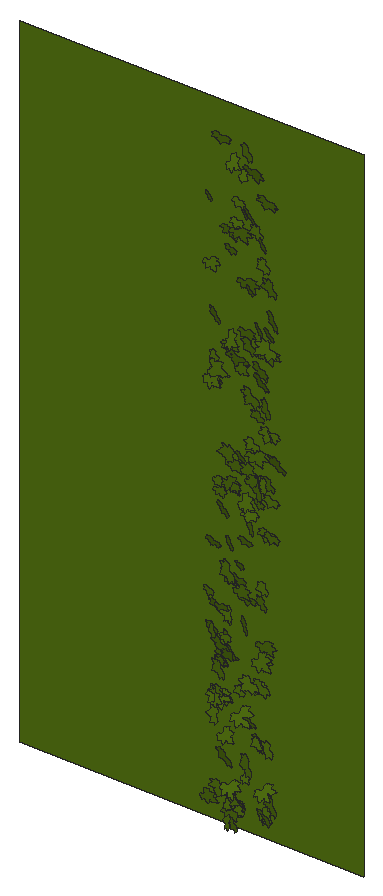
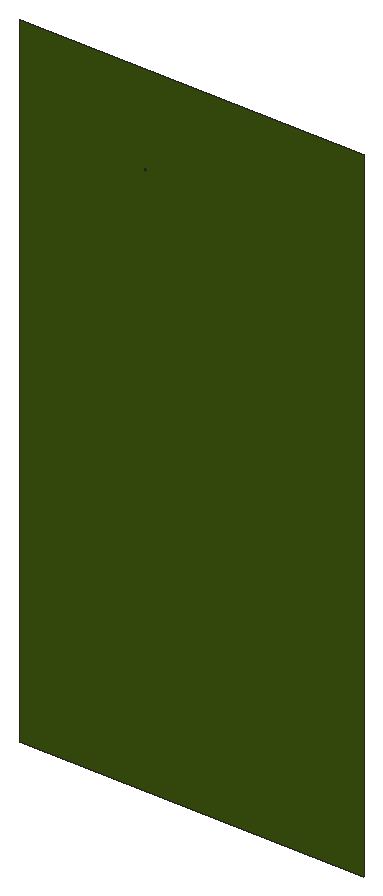
# SketchUp Ruby script. Lengths in inches.
U = 1.inch
M = Sketchup.active_model
def pt(a) = Geom::Point3d.new(a.map { |v| v * U })
def face(e, loops, mat)
  f = e.add_face(loops[0].map { |a| pt(a) })
  loops[1..].each { |l| e.add_face(l.map { |a| pt(a) }).erase! }
  f.material = f.back_material = mat if mat
  f
end
# faces: each face lists its corners as indices into pts; further lists are holes
def faces(e, pts, list, mat = nil) = list.each { |f| face(e, (f[0].is_a?(Array) ? f : [f]).map { |l| l.map { |i| pts[i] } }, mat) }
# xy, xz, yz: faces in a plane at the given z, y or x. An outline is a flat list of corners, or four numbers for a rectangle; further outlines are holes
def ring(l) = l.size == 4 ? [[l[0], l[1]], [l[2], l[1]], [l[2], l[3]], [l[0], l[3]]] : l.each_slice(2).to_a
def flat(e, list, mat, &to3) = list.each { |f| face(e, (f[0].is_a?(Array) ? f : [f]).map { |l| ring(l).map { |u, v| to3.(u, v) } }, mat) }
def xy(e, z, list, mat = nil) = flat(e, list, mat) { |x, y| [x, y, z] }
def xz(e, y, list, mat = nil) = flat(e, list, mat) { |x, z| [x, y, z] }
def yz(e, x, list, mat = nil) = flat(e, list, mat) { |y, z| [x, y, z] }
def lines(e, pts, list) = list.each { |a, b| e.add_line(pt(pts[a]), pt(pts[b])) }
# prism: a flat outline (further loops are holes) pulled along v
def prism(e, loops, v, mat = nil)
  f = face(e, loops, mat); d = Geom::Vector3d.new(v.map { |x| x * U })
  f.pushpull(f.normal.samedirection?(d) ? d.length : -d.length)
end
def box(e, o, s, mat = nil) = prism(e, [[o, [o[0] + s[0], o[1], o[2]], [o[0] + s[0], o[1] + s[1], o[2]], [o[0], o[1] + s[1], o[2]]]], [0, 0, s[2]], mat)
def at(x, y, z, deg = 0) = Geom::Transformation.translation(pt([x, y, z])) * Geom::Transformation.rotation(ORIGIN, Z_AXIS, deg.degrees)
def axes(o, x, y, z) = Geom::Transformation.new([*x, 0, *y, 0, *z, 0, *pt(o).to_a, 1])
def part(name) = M.definitions.add(name)
# library, detail: a bought-in or finely detailed component or shape, given as its bounding box
def library(name, o, s) = part(name).tap { |d| box(d.entities, o, s) }
def detail(e, o, s) = box(e.add_group.entities, o, s)
def put(e, d, t, mat = nil) = e.add_instance(d, t).tap { |i| i.material = mat if mat }
def group(e, t, mat = nil) = e.add_group.tap { |g| g.transformation = t; g.material = mat if mat }.entities
root = M.entities
M.materials.add("[Vegetation Blur 03]").color = [83, 114, 18]
c1 = part("ivy")
xy(c1.entities,0,[[0.782,0,0.786,0,0.787,0.005,0.789,0.009,0.821,0.072,0.875,0.147,1.001,0.272,1.073,0.331,1.137,0.363,1.178,0.379,1.223,0.384,1.272,0.383,1.311,0.374,1.36,0.355,1.399,0.334,1.491,0.285,1.541,0.244,1.583,0.199,1.617,0.15,1.64,0.128,1.662,0.115,1.717,0.105,1.745,0.093,1.784,0.054,1.819,0.057,1.854,0.064,1.882,0.075,1.896,0.074,1.91,0.071,1.937,0.063,1.964,0.053,1.99,0.038,2.016,0.015,2.034,0.002,2.04,0,2.038,0.003,2.036,0.007,2.033,0.038,2.036,0.068,2.045,0.1,2.055,0.116,2.064,0.123,2.077,0.129,2.088,0.129,2.106,0.132,2.118,0.13,2.179,0.132,2.207,0.133,2.225,0.133,2.242,0.138,2.22,0.162,2.207,0.186,2.206,0.213,2.212,0.236,2.228,0.262,2.247,0.274,2.298,0.283,2.355,0.294,2.37,0.296,2.376,0.295,2.377,0.3,2.377,0.303,2.385,0.329,2.411,0.37,2.426,0.392,2.449,0.407,2.511,0.426,2.561,0.444,2.619,0.466,2.589,0.469,2.561,0.476,2.501,0.5,2.449,0.516,2.424,0.523,2.401,0.535,2.377,0.556,2.372,0.568,2.36,0.575,2.268,0.586,2.225,0.592,2.207,0.599,2.194,0.61,2.143,0.65,2.13,0.664,2.122,0.682,2.123,0.7,2.13,0.719,2.148,0.75,2.17,0.781,2.195,0.807,2.221,0.828,2.284,0.874,2.291,0.88,2.288,0.887,2.276,0.9,2.267,0.916,2.265,0.933,2.273,0.967,2.292,1.002,2.313,1.03,2.334,1.054,2.348,1.067,2.358,1.074,2.363,1.076,2.362,1.081,2.35,1.094,2.347,1.11,2.35,1.143,2.359,1.18,2.385,1.254,2.415,1.324,2.448,1.393,2.45,1.4,2.446,1.398,2.44,1.394,2.427,1.383,2.402,1.36,2.376,1.339,2.345,1.324,2.305,1.309,2.282,1.303,2.273,1.306,2.245,1.294,2.212,1.287,2.187,1.291,2.163,1.301,2.142,1.316,2.134,1.327,2.124,1.325,2.09,1.292,2.053,1.259,2.014,1.234,1.973,1.215,1.954,1.21,1.931,1.208,1.909,1.212,1.893,1.22,1.879,1.233,1.872,1.248,1.867,1.281,1.864,1.319,1.821,1.258,1.773,1.197,1.726,1.141,1.698,1.121,1.679,1.116,1.666,1.117,1.647,1.122,1.632,1.129,1.62,1.141,1.617,1.154,1.617,1.219,1.621,1.254,1.623,1.268,1.623,1.281,1.618,1.314,1.606,1.346,1.603,1.375,1.607,1.403,1.603,1.467,1.599,1.499,1.605,1.525,1.614,1.552,1.629,1.577,1.635,1.589,1.629,1.587,1.618,1.582,1.596,1.566,1.581,1.556,1.568,1.552,1.557,1.55,1.545,1.553,1.531,1.562,1.522,1.572,1.504,1.591,1.486,1.611,1.474,1.631,1.457,1.666,1.455,1.684,1.457,1.698,1.452,1.715,1.444,1.728,1.424,1.754,1.419,1.772,1.423,1.786,1.434,1.819,1.444,1.848,1.446,1.855,1.44,1.861,1.43,1.867,1.386,1.904,1.349,1.948,1.326,1.973,1.31,1.995,1.288,2.048,1.284,2.153,1.287,2.254,1.284,2.255,1.282,2.253,1.278,2.247,1.274,2.237,1.266,2.216,1.226,2.125,1.208,2.076,1.184,2.033,1.155,1.984,1.135,1.942,1.111,1.899,1.083,1.861,1.053,1.85,1.059,1.83,1.061,1.809,1.056,1.79,1.049,1.767,1.04,1.749,1.018,1.733,0.994,1.726,0.942,1.734,0.95,1.6875,0.944,1.645,0.932,1.608,0.911,1.585,0.881,1.58,0.854,1.582,0.828,1.588,0.785,1.618,0.773,1.625,0.775,1.614,0.779,1.598,0.796,1.502,0.818,1.402,0.861,1.283,0.882,1.224,0.894,1.174,0.892,1.148,0.886,1.123,0.881,1.107,0.872,1.099,0.849,1.094,0.818,1.092,0.789,1.098,0.762,1.107,0.753,1.113,0.721,1.139,0.698,1.163,0.678,1.194,0.665,1.224,0.628,1.28,0.612,1.312,0.606,1.327,0.606,1.314,0.599,1.282,0.594,1.267,0.581,1.256,0.544,1.245,0.512,1.244,0.473,1.249,0.444,1.256,0.382,1.288,0.339,1.306,0.324,1.316,0.317,1.324,0.309,1.326,0.27,1.314,0.227,1.313,0.185,1.3125,0.152,1.317,0.122,1.328,0.092,1.345,0.073,1.353,0.079,1.338,0.092,1.308,0.117,1.249,0.13,1.215,0.139,1.164,0.147,1.148,0.157,1.136,0.163,1.122,0.174,1.086,0.177,1.067,0.182,1.054,0.186,1.043,0.191,1.038,0.211,1.028,0.237,1.005,0.25,0.974,0.253,0.96,0.25,0.944,0.242,0.914,0.243,0.906,0.249,0.902,0.26,0.894,0.289,0.88,0.307,0.873,0.322,0.862,0.364,0.799,0.403,0.738,0.431,0.709,0.439,0.691,0.441,0.678,0.4375,0.66,0.428,0.645,0.394,0.623,0.303,0.594,0.255,0.581,0.214,0.577,0.179,0.573,0.173,0.568,0.175,0.561,0.167,0.55,0.141,0.523,0.113,0.503,0.077,0.49,0.045,0.486,0.026,0.485,0.019,0.486,0.011,0.483,0,0.471,0.014,0.467,0.044,0.455,0.058,0.447,0.07,0.438,0.097,0.411,0.125,0.394,0.158,0.377,0.174,0.366,0.182,0.359,0.185,0.361,0.242,0.331,0.253,0.316,0.258,0.303,0.262,0.283,0.274,0.278,0.308,0.274,0.341,0.252,0.366,0.226,0.366,0.222,0.37,0.22,0.38,0.221,0.395,0.221,0.425,0.216,0.45,0.207,0.465,0.192,0.473,0.178,0.484,0.15,0.489,0.116,0.483,0.089,0.468,0.058,0.45,0.035,0.435,0.018,0.429,0.011,0.434,0.012,0.438,0.014,0.469,0.019,0.542,0.016,0.581,0.015,0.612,0.027,0.68,0.055,0.696,0.057,0.712,0.052,0.73,0.045,0.741,0.036,0.766,0.014]])
xz(root,174.5,[[10,5,34.46,51]],"[Vegetation Blur 03]")
put(root,c1,axes([24.22,173.7,18.05],[0.16976,0.07158,-0.29867],[-0.3654,0.12339,-0.13369],[-0.04012,-0.82092,-0.04613]),"[Vegetation Blur 03]")
put(root,c1,axes([23.86,173.7,45.46],[0.26677,-0.13263,-0.08131],[-0.08808,0.11667,-0.22242],[-0.07951,-0.57427,-0.02641]),"[Vegetation Blur 03]")
put(root,c1,axes([23.73,173.7,20.28],[0.33233,-0.0945,-0.02615],[-0.02986,0.03657,-0.27359],[-0.04737,-0.68607,-0.01098]),"[Vegetation Blur 03]")
put(root,c1,axes([24.45,173.7,38.07],[0.15729,0.04975,-0.38701],[-0.46067,0.26502,-0.11935],[-0.11503,-0.99334,-0.05122]),"[Vegetation Blur 03]")
put(root,c1,axes([23.96,173.7,23.48],[0.35115,0.05857,-0.18722],[-0.23024,0.1649,-0.27952],[-0.02054,-0.84722,-0.06735]),"[Vegetation Blur 03]")
put(root,c1,axes([23.33,173.7,6.55],[0.26007,-0.08689,0.38147],[0.46915,0.07766,-0.21026],[0.0126,-1.09796,-0.04506]),"[Vegetation Blur 03]")
put(root,c1,axes([24.38,173.7,19.54],[0.17674,0.08976,-0.26223],[-0.3229,0.11764,-0.13863],[-0.02967,-0.7454,-0.05345]),"[Vegetation Blur 03]")
put(root,c1,axes([24.66,173.7,34.0625],[0.08767,0.08949,-0.34433],[-0.41588,0.19217,-0.06267],[-0.08326,-0.86566,-0.04951]),"[Vegetation Blur 03]")
put(root,c1,axes([24.3,173.7,18.08],[0.25432,-0.19046,-0.24423],[-0.28944,0.16036,-0.22043],[-0.11975,-0.79207,0.0141]),"[Vegetation Blur 03]")
put(root,c1,axes([23.53,173.7,40.9],[0.40459,0.02303,0.19859],[0.2435,-0.01333,-0.3302],[0.00625,-0.97145,0.00924]),"[Vegetation Blur 03]")
put(root,c1,axes([24.73,173.7,12.75],[0.10121,-0.15146,-0.36108],[-0.44341,0.10659,-0.08981],[-0.06746,-0.92784,0.04863]),"[Vegetation Blur 03]")
put(root,c1,axes([24.4375,173.7,35.5],[0.20022,-0.05357,-0.19807],[-0.24233,0.03356,-0.1646],[-0.02917,-0.64656,0.00787]),"[Vegetation Blur 03]")
put(root,c1,axes([24.75,173.7,14.2],[0.11196,0.05174,-0.31654],[-0.38834,-0.01941,-0.09199],[0.01605,-0.83049,-0.01757]),"[Vegetation Blur 03]")
put(root,c1,axes([23.51,173.7,33.24],[0.28098,0.0713,0.44477],[0.5442,-0.14112,-0.22543],[-0.04527,-1.25382,0.05067]),"[Vegetation Blur 03]")
put(root,c1,axes([24.04,173.7,12.81],[0.09158,0.04301,0.34718],[0.42504,-0.06647,-0.07338],[-0.02723,-0.89296,0.02219]),"[Vegetation Blur 03]")
put(root,c1,axes([24.68,173.7,15.93],[0.35185,-0.14327,-0.37157],[-0.44566,0.19161,-0.29272],[-0.11623,-1.16844,-0.00244]),"[Vegetation Blur 03]")
put(root,c1,axes([24.55,173.7,14.13],[0.45581,0.11699,-0.31525],[-0.38742,-0.0162,-0.37405],[0.04848,-1.22937,-0.02507]),"[Vegetation Blur 03]")
put(root,c1,axes([24.43,173.7,17.4],[0.54219,-0.07189,-0.27942],[-0.3337,0.21166,-0.43986],[-0.08416,-1.30245,-0.05606]),"[Vegetation Blur 03]")
put(root,c1,axes([24.3,173.7,49.41],[0.46012,0.08661,-0.09796],[-0.12471,0.12465,-0.37281],[0.02504,-0.97055,-0.05662]),"[Vegetation Blur 03]")
put(root,c1,axes([24.28,173.7,8.16],[0.58678,0.063,-0.19417],[-0.23912,0.05083,-0.47872],[0.01906,-1.30195,-0.02809]),"[Vegetation Blur 03]")
put(root,c1,axes([23.79,173.7,13.53],[0.59488,0.11123,0.16598],[0.20655,-0.0688,-0.48585],[0.04022,-1.29188,0.04016]),"[Vegetation Blur 03]")
put(root,c1,axes([24.82,173.7,16.17],[0.24584,0.04332,-0.24097],[-0.29547,0.08344,-0.19842],[-0.01781,-0.78621,-0.03434]),"[Vegetation Blur 03]")
put(root,c1,axes([24.92,173.7,10.26],[0.33588,0.02262,-0.39753],[-0.47681,0.26549,-0.26596],[-0.10014,-1.18823,-0.067]),"[Vegetation Blur 03]")
put(root,c1,axes([23.96,173.7,33.59],[0.09221,0.01276,0.54145],[0.66339,-0.02223,-0.07517],[-0.00985,-1.37816,0.00623]),"[Vegetation Blur 03]")
put(root,c1,axes([24.26,173.7,27.17],[0.25,-0.03131,0.17773],[0.21716,-0.03407,-0.2044],[-0.02234,-0.68141,0.00205]),"[Vegetation Blur 03]")
put(root,c1,axes([24.7,173.7,16.5625],[0.39633,-0.13888,-0.234],[-0.27566,0.17367,-0.32719],[-0.1038,-0.99151,-0.02453]),"[Vegetation Blur 03]")
put(root,c1,axes([24.28,173.7,26.63],[0.3534,-0.02851,0.14206],[0.17452,0.03242,-0.28817],[-0.00545,-0.81,-0.01653]),"[Vegetation Blur 03]")
put(root,c1,axes([24.72,173.7,26.03],[0.4235,-0.13743,-0.21645],[-0.24668,0.24247,-0.3457],[-0.1181,-0.99928,-0.05411]),"[Vegetation Blur 03]")
put(root,c1,axes([24.5,173.7,15.86],[0.26031,-0.0805,0.12545],[0.1556,0.01165,-0.21388],[-0.03078,-0.62197,-0.02024]),"[Vegetation Blur 03]")
put(root,c1,axes([24.36,173.7,19.28],[0.41549,-0.08208,0.11963],[0.15106,0.12998,-0.33542],[-0.01613,-0.89729,-0.05953]),"[Vegetation Blur 03]")
put(root,c1,axes([25.36,173.7,17.78],[0.07952,-0.02515,-0.25316],[-0.29832,0.17612,-0.06516],[-0.08589,-0.63499,-0.00805]),"[Vegetation Blur 03]")
put(root,c1,axes([25.77,173.7,29.72],[0.10377,0.02186,-0.53621],[-0.65451,0.12482,-0.08356],[-0.05827,-1.36305,-0.01625]),"[Vegetation Blur 03]")
put(root,c1,axes([25.57,173.7,18.94],[0.04974,-0.00028,-0.27725],[-0.32677,0.19308,-0.03908],[-0.09286,-0.67961,-0.01099]),"[Vegetation Blur 03]")
put(root,c1,axes([25.65,173.7,19.46],[0.08632,-0.07212,-0.36138],[-0.4424,0.06914,-0.07256],[-0.03977,-0.92577,0.02273]),"[Vegetation Blur 03]")
put(root,c1,axes([25.34,173.7,22.4375],[0.39881,-0.16855,-0.40776],[-0.49292,0.16963,-0.33214],[-0.11562,-1.30452,0.00949]),"[Vegetation Blur 03]")
put(root,c1,axes([25.57,173.7,6.12],[0.10497,-0.16799,-0.28426],[-0.34085,0.17977,-0.10055],[-0.10859,-0.72666,0.04084]),"[Vegetation Blur 03]")
put(root,c1,axes([24.83,173.7,17.5625],[0.3425,-0.04443,0.04433],[0.05384,-0.01893,-0.28004],[-0.02276,-0.71335,0.00467]),"[Vegetation Blur 03]")
put(root,c1,axes([25.46,173.7,23.85],[0.19183,-0.05588,-0.2698],[-0.31224,0.23474,-0.15552],[-0.11192,-0.75067,-0.02855]),"[Vegetation Blur 03]")
put(root,c1,axes([24.54,173.7,10.75],[0.24435,0.09355,0.35761],[0.44053,-0.04867,-0.19849],[0.00137,-1.03125,0.04181]),"[Vegetation Blur 03]")
put(root,c1,axes([25.06,173.7,6.54],[0.09713,0.02395,0.23937],[0.28996,-0.10667,-0.07669],[-0.04564,-0.62678,0.0222]),"[Vegetation Blur 03]")
put(root,c1,axes([24.87,173.7,36.24],[0.48068,0.01776,0.03152],[0.03794,0.06838,-0.39147],[0.01124,-0.98997,-0.02647]),"[Vegetation Blur 03]")
put(root,c1,axes([24.84,173.7,6.32],[0.46585,0.02288,0.14137],[0.17091,0.11775,-0.37813],[0.0303,-1.01595,-0.04064]),"[Vegetation Blur 03]")
put(root,c1,axes([25.4,173.7,17.05],[0.36602,-0.17334,-0.17958],[-0.2031,0.19186,-0.30487],[-0.11941,-0.85763,-0.0319]),"[Vegetation Blur 03]")
put(root,c1,axes([24.8,173.7,43.67],[0.63593,0.00439,0.02808],[0.0337,0.19557,-0.51321],[0.00724,-1.29586,-0.07736]),"[Vegetation Blur 03]")
put(root,c1,axes([25.23,173.7,42.55],[0.37054,-0.08411,-0.02834],[-0.02969,0.09383,-0.30232],[-0.04467,-0.76008,-0.03419]),"[Vegetation Blur 03]")
put(root,c1,axes([24.77,173.7,7.84],[0.46596,0.12424,0.22352],[0.28037,-0.18097,-0.37349],[0.00652,-1.09739,0.0869]),"[Vegetation Blur 03]")
put(root,c1,axes([25.11,173.7,21.06],[0.25004,-0.05522,0.19659],[0.24228,0.07618,-0.20189],[0.00655,-0.71038,-0.03693]),"[Vegetation Blur 03]")
put(root,c1,axes([25.61,173.7,7.81],[0.43018,0.03461,-0.33433],[-0.40999,0.03807,-0.35076],[-0.00059,-1.2218,-0.0204]),"[Vegetation Blur 03]")
put(root,c1,axes([25.03,173.7,16.03],[0.13975,-0.17275,0.35559],[0.44281,0.11446,-0.10717],[0.0284,-0.9346,-0.07885]),"[Vegetation Blur 03]")
put(root,c1,axes([25.09,173.7,35.97],[0.08788,0.15958,0.41108],[0.50211,-0.20702,-0.05886],[-0.08717,-1.03158,0.0754]),"[Vegetation Blur 03]")
put(root,c1,axes([24.69,173.7,27.21],[0.49372,-0.08066,0.3359],[0.41334,0.06825,-0.4021],[-0.00879,-1.32093,-0.04129]),"[Vegetation Blur 03]")
put(root,c1,axes([25.59,173.7,6.14],[0.34936,-0.1754,-0.17065],[-0.20005,0.12722,-0.29335],[-0.10473,-0.82812,-0.00892]),"[Vegetation Blur 03]")
put(root,c1,axes([25.42,173.7,27.82],[0.46927,-0.11869,-0.14311],[-0.17217,0.07416,-0.3857],[-0.06659,-1.02821,-0.0113]),"[Vegetation Blur 03]")
put(root,c1,axes([25.33,173.7,35.9375],[0.61818,0.02753,-0.20694],[-0.25253,0.20999,-0.49806],[-0.0265,-1.35881,-0.08116]),"[Vegetation Blur 03]")
put(root,c1,axes([25.19,173.7,47.34],[0.1221,0.15901,0.36769],[0.45566,-0.11863,-0.09271],[-0.03634,-0.95319,0.07288]),"[Vegetation Blur 03]")
put(root,c1,axes([25.49,173.7,7.77],[0.53938,-0.11783,-0.24861],[-0.28048,0.34993,-0.43141],[-0.13192,-1.22575,-0.09926]),"[Vegetation Blur 03]")
put(root,c1,axes([26.39,173.7,45.38],[0.10747,0.09693,-0.42949],[-0.50045,0.37307,-0.07017],[-0.16944,-1.0404,-0.06517]),"[Vegetation Blur 03]")
put(root,c1,axes([25.73,173.7,44.4],[0.32282,0.01218,-0.05233],[-0.06347,-0.05325,-0.26277],[0.01083,-0.67519,0.01978]),"[Vegetation Blur 03]")
put(root,c1,axes([25.32,173.7,28.54],[0.35919,-0.07581,0.24051],[0.29623,0.02355,-0.29351],[-0.02119,-0.9558,-0.02631]),"[Vegetation Blur 03]")
put(root,c1,axes([25.9,173.7,45.8],[0.32239,-0.01176,-0.10948],[-0.13423,-0.01041,-0.2631],[-0.00333,-0.71849,0.00561]),"[Vegetation Blur 03]")
put(root,c1,axes([26.41,173.7,7.01],[0.06839,0.01536,-0.24268],[-0.29667,-0.04173,-0.0561],[0.02144,-0.62648,-0.00221]),"[Vegetation Blur 03]")
put(root,c1,axes([26.32,173.7,14.71],[0.15181,-0.00524,-0.23084],[-0.28286,-0.00517,-0.12389],[0.00101,-0.66057,0.0028]),"[Vegetation Blur 03]")
put(root,c1,axes([26.65,173.7,18.9],[0.06026,0.01776,-0.40154],[-0.46093,0.35917,-0.04358],[-0.17229,-0.95467,-0.02387]),"[Vegetation Blur 03]")
put(root,c1,axes([26.08,173.7,29.6],[0.28037,-0.06157,-0.15463],[-0.18018,0.15229,-0.22714],[-0.06579,-0.67947,-0.0369]),"[Vegetation Blur 03]")
put(root,c1,axes([25.68,173.7,21.7],[0.47998,-0.11829,-0.01678],[-0.01365,0.11877,-0.39191],[-0.0595,-0.98146,-0.0454]),"[Vegetation Blur 03]")
put(root,c1,axes([25.9,173.7,22.55],[0.3065,-0.10801,0.00878],[0.01921,0.10156,-0.25024],[-0.05001,-0.62289,-0.04232]),"[Vegetation Blur 03]")
put(root,c1,axes([25.36,173.7,43.53],[0.56255,-0.01811,0.20546],[0.25121,0.13405,-0.45628],[0.01862,-1.26114,-0.05145]),"[Vegetation Blur 03]")
put(root,c1,axes([26.37,173.7,24.24],[0.26692,0.10027,-0.19485],[-0.24358,0.09015,-0.21495],[0.00657,-0.73139,-0.05321]),"[Vegetation Blur 03]")
put(root,c1,axes([25.41,173.7,12.34],[0.39393,0.1891,0.39235],[0.48905,-0.10099,-0.3194],[0.01969,-1.27498,0.08349]),"[Vegetation Blur 03]")
put(root,c1,axes([25.85,173.7,34.7],[0.23197,-0.0436,0.29061],[0.3566,0.00644,-0.18945],[-0.00894,-0.8745,-0.01588]),"[Vegetation Blur 03]")
put(root,c1,axes([26.79,173.7,10.44],[0.28462,-0.17247,-0.45638],[-0.54186,0.28495,-0.24203],[-0.16158,-1.25936,0.00774]),"[Vegetation Blur 03]")
put(root,c1,axes([25.66,173.7,20.58],[0.39343,-0.07208,0.30532],[0.37571,0.06003,-0.32024],[-0.0052,-1.11557,-0.03696]),"[Vegetation Blur 03]")
put(root,c1,axes([26.15,173.7,46.95],[0.0888,0.09674,0.25308],[0.31076,-0.1168,-0.0656],[-0.0424,-0.6534,0.0492]),"[Vegetation Blur 03]")
put(root,c1,axes([27.1,173.7,29.1],[0.14596,0.116,-0.44941],[-0.55223,-0.05004,-0.12149],[0.03805,-1.17121,-0.03932]),"[Vegetation Blur 03]")
put(root,c1,axes([26.33,173.7,20.51],[0.38415,0.08832,-0.09325],[-0.11924,0.10565,-0.31143],[0.02608,-0.81794,-0.0503]),"[Vegetation Blur 03]")
put(root,c1,axes([26.58,173.7,45.38],[0.42548,-0.09437,-0.33716],[-0.38139,0.39508,-0.33797],[-0.16527,-1.15464,-0.08808]),"[Vegetation Blur 03]")
put(root,c1,axes([26.65,173.7,49.45],[0.35368,-0.15187,-0.29343],[-0.34945,0.17479,-0.29479],[-0.11221,-1.02299,-0.00681]),"[Vegetation Blur 03]")
put(root,c1,axes([26.77,173.7,12.8],[0.21856,0.08137,-0.22546],[-0.27868,0.10188,-0.17416],[-0.01478,-0.71768,-0.05028]),"[Vegetation Blur 03]")
put(root,c1,axes([26.24,173.7,8.72],[0.17985,0.03398,0.21034],[0.25744,-0.07475,-0.14472],[-0.02044,-0.64238,0.02797]),"[Vegetation Blur 03]")
put(root,c1,axes([26.74,173.7,37.11],[0.38374,-0.03816,-0.34105],[-0.41282,0.15382,-0.31209],[-0.06752,-1.15732,-0.03024]),"[Vegetation Blur 03]")
put(root,c1,axes([27.11,173.7,25.25],[0.07886,-0.02245,-0.3122],[-0.36365,0.24601,-0.06396],[-0.11923,-0.76517,-0.0114]),"[Vegetation Blur 03]")
put(root,c1,axes([26.05,173.7,25.98],[0.16307,0.08475,0.41488],[0.5096,-0.07153,-0.13111],[-0.02064,-1.09626,0.04063]),"[Vegetation Blur 03]")
put(root,c1,axes([26.67,173.7,15.56],[0.42678,-0.01115,-0.26433],[-0.32354,-0.0687,-0.34749],[0.01587,-1.10035,0.02437]),"[Vegetation Blur 03]")
put(root,c1,axes([26.07,173.7,37.48],[0.51847,-0.08238,0.09913],[0.12469,0.09368,-0.42215],[-0.02842,-1.09178,-0.0437]),"[Vegetation Blur 03]")
put(root,c1,axes([25.88,173.7,40.53],[0.5764,-0.04158,0.19028],[0.23362,0.17732,-0.46527],[0.01378,-1.26714,-0.07135]),"[Vegetation Blur 03]")
put(root,c1,axes([26.73,173.7,40.41],[0.29856,-0.10941,-0.11062],[-0.12269,0.1536,-0.24445],[-0.0784,-0.65702,-0.03873]),"[Vegetation Blur 03]")
put(root,c1,axes([26.68,173.7,34.02],[0.54012,-0.12372,-0.29412],[-0.3556,0.12595,-0.44329],[-0.0839,-1.33021,-0.01462]),"[Vegetation Blur 03]")
put(root,c1,axes([26.51,173.7,26.15],[0.44019,0.01869,-0.05575],[-0.06711,-0.08998,-0.3577],[0.01564,-0.91223,0.03414]),"[Vegetation Blur 03]")
put(root,c1,axes([26.97,173.7,30.82],[0.32974,-0.02071,-0.22461],[-0.27537,-0.01528,-0.26905],[-0.00296,-0.88368,0.00992]),"[Vegetation Blur 03]")
put(root,c1,axes([27.55,173.7,32.67],[0.16409,0.0678,-0.30247],[-0.37206,0.03564,-0.13319],[-0.00256,-0.83328,-0.0303]),"[Vegetation Blur 03]")
put(root,c1,axes([26.54,173.7,27.74],[0.26787,-0.06927,0.33281],[0.40897,0.07748,-0.21671],[0.01312,-1.00101,-0.0398]),"[Vegetation Blur 03]")
put(root,c1,axes([26.39,173.7,47.96],[0.62307,-0.149,0.09151],[0.12235,0.19755,-0.50432],[-0.05332,-1.28769,-0.08796]),"[Vegetation Blur 03]")
put(root,c1,axes([27.46,173.7,11.95],[0.28434,-0.07307,-0.35446],[-0.41994,0.239,-0.23213],[-0.11635,-1.04116,-0.02841]),"[Vegetation Blur 03]")
put(root,c1,axes([27.55,173.7,44.49],[0.19509,-0.01615,-0.32843],[-0.40182,0.04546,-0.15934],[-0.0233,-0.91916,-0.00211]),"[Vegetation Blur 03]")
put(root,c1,axes([27.5,173.7,28.49],[0.3874,-0.28987,-0.42046],[-0.49062,0.32448,-0.33628],[-0.21109,-1.28615,0.00992]),"[Vegetation Blur 03]")
put(root,c1,axes([27.53,173.7,11.82],[0.20749,-0.03484,-0.23563],[-0.28917,-0.01288,-0.16931],[-0.00479,-0.73151,0.0142]),"[Vegetation Blur 03]")
put(root,c1,axes([26.54,173.7,29.65],[0.54429,0.0275,0.19656],[0.23996,0.06284,-0.44397],[0.02457,-1.22318,-0.01839]),"[Vegetation Blur 03]")
put(root,c1,axes([27.9,173.7,20.83],[0.12874,0.00958,-0.35889],[-0.43298,0.16781,-0.10275],[-0.07698,-0.92784,-0.02229]),"[Vegetation Blur 03]")
put(root,c1,axes([27.39,173.7,35.04],[0.44147,-0.0788,-0.2903],[-0.33877,0.28169,-0.35517],[-0.11502,-1.13213,-0.06817]),"[Vegetation Blur 03]")
put(root,c1,axes([27.3125,173.7,26.97],[0.32248,-0.05987,-0.04087],[-0.04757,0.05862,-0.26354],[-0.03303,-0.669,-0.01944]),"[Vegetation Blur 03]")
put(root,c1,axes([27.38,173.7,38.23],[0.34481,-0.20074,-0.10306],[-0.10927,0.15385,-0.29065],[-0.11628,-0.7398,-0.03248]),"[Vegetation Blur 03]")
put(root,c1,axes([27.41,173.7,15.59],[0.47072,-0.03676,-0.23219],[-0.28418,0.02801,-0.38445],[-0.02233,-1.13149,-0.00197]),"[Vegetation Blur 03]")
put(root,c1,axes([27.98,173.7,21.86],[0.16539,-0.02327,-0.29289],[-0.35869,0.02592,-0.13523],[-0.01618,-0.81273,0.00407]),"[Vegetation Blur 03]")
put(root,c1,axes([27.24,173.7,35.81],[0.56634,-0.19077,-0.13861],[-0.15859,0.16167,-0.4666],[-0.11086,-1.2059,-0.04063]),"[Vegetation Blur 03]")
put(root,c1,axes([27.27,173.7,14.78],[0.17104,0.07406,0.23051],[0.28468,-0.03259,-0.13906],[0.00499,-0.6787,0.03183]),"[Vegetation Blur 03]")
put(root,c1,axes([28.125,173.7,28.4375],[0.12105,-0.13191,-0.28197],[-0.3442,0.10689,-0.10629],[-0.07075,-0.74572,0.03464]),"[Vegetation Blur 03]")
put(root,c1,axes([27.97,173.7,42.55],[0.26106,-0.06742,-0.29363],[-0.35973,0.03582,-0.21432],[-0.03335,-0.91402,0.01326]),"[Vegetation Blur 03]")
put(root,c1,axes([27.59,173.7,43.82],[0.38591,-0.21569,-0.14541],[-0.15737,0.19687,-0.32414],[-0.13402,-0.85224,-0.03808]),"[Vegetation Blur 03]")
put(root,c1,axes([28.3,173.7,28.625],[0.1471,0.09742,-0.39347],[-0.48397,0.0748,-0.1176],[-0.02114,-1.03455,-0.04555]),"[Vegetation Blur 03]")
put(root,c1,axes([26.95,173.7,16.35],[0.3582,0.03063,0.42978],[0.52659,-0.05959,-0.29166],[-0.01559,-1.30923,0.02333]),"[Vegetation Blur 03]")
put(root,c1,axes([27.29,173.7,16.62],[0.36162,0.06548,0.17991],[0.22033,0.0215,-0.29621],[0.03262,-0.87124,0.00621]),"[Vegetation Blur 03]")
put(root,c1,axes([28.09,173.7,37.49],[0.37878,0.01189,-0.41383],[-0.50562,-0.09055,-0.30867],[0.03871,-1.29927,0.01773]),"[Vegetation Blur 03]")
put(root,c1,axes([27.61,173.7,46.52],[0.51764,0.02568,-0.18283],[-0.22378,0.14257,-0.41887],[-0.01616,-1.15189,-0.05592]),"[Vegetation Blur 03]")
put(root,c1,axes([27.53,173.7,7.34],[0.50401,-0.18357,-0.11952],[-0.1351,0.15116,-0.41597],[-0.10561,-1.06941,-0.03828]),"[Vegetation Blur 03]")
put(root,c1,axes([27.13,173.7,8.1],[0.37101,0.18964,0.31894],[0.39968,-0.06988,-0.30314],[0.03834,-1.10666,0.0738]),"[Vegetation Blur 03]")
put(root,c1,axes([28.46,173.7,41.29],[0.18125,0.04011,-0.45454],[-0.55361,0.15105,-0.14494],[-0.06386,-1.19573,-0.03356]),"[Vegetation Blur 03]")
put(root,c1,axes([28.0625,173.7,33.625],[0.34504,-0.21965,-0.31495],[-0.37042,0.22285,-0.29474],[-0.152,-1.04167,0.00335]),"[Vegetation Blur 03]")
put(root,c1,axes([28.31,173.7,11.85],[0.21313,-0.07118,-0.35531],[-0.43534,0.04461,-0.17534],[-0.03471,-0.99647,0.01753]),"[Vegetation Blur 03]")
put(root,c1,axes([28.11,173.7,38.11],[0.28115,-0.04858,-0.24392],[-0.28246,0.2397,-0.22437],[-0.10049,-0.80964,-0.05179]),"[Vegetation Blur 03]")
put(root,c1,axes([27.71,173.7,25.31],[0.48743,0.04761,-0.1367],[-0.16843,0.04371,-0.39762],[0.01495,-1.05971,-0.02254]),"[Vegetation Blur 03]")
put(root,c1,axes([28.15,173.7,31.74],[0.24639,-0.0769,-0.23479],[-0.27054,0.21951,-0.20041],[-0.10474,-0.7479,-0.03468]),"[Vegetation Blur 03]")
put(root,c1,axes([28.43,173.7,8.45],[0.27997,-0.09905,-0.45822],[-0.54252,0.30141,-0.23104],[-0.15235,-1.25535,-0.01932]),"[Vegetation Blur 03]")
put(root,c1,axes([27.3,173.7,36.5],[0.59787,0.07047,0.08314],[0.09735,0.14687,-0.48587],[0.04553,-1.23935,-0.05285]),"[Vegetation Blur 03]")
put(root,c1,axes([27.25,173.7,17.73],[0.50143,-0.04661,0.23263],[0.28578,0.12116,-0.40648],[0.00953,-1.18071,-0.05089]),"[Vegetation Blur 03]")
put(root,c1,axes([27.58,173.7,6.72],[0.18512,0.00647,0.33943],[0.41367,-0.0999,-0.14998],[-0.04308,-0.93144,0.01844]),"[Vegetation Blur 03]")
put(root,c1,axes([27.88,173.7,31.85],[0.50815,0.02983,-0.17456],[-0.21367,-0.02159,-0.41487],[0.01743,-1.13431,0.00331]),"[Vegetation Blur 03]")
put(root,c1,axes([28.89,173.7,30.04],[0.15268,0.21133,-0.48982],[-0.60568,0.18355,-0.11329],[-0.06257,-1.26109,-0.09857]),"[Vegetation Blur 03]")
put(root,c1,axes([28.09,173.7,27.5],[0.38921,0.02788,-0.11804],[-0.14492,0.01541,-0.31769],[0.01009,-0.85429,-0.00958]),"[Vegetation Blur 03]")
put(root,c1,axes([28.43,173.7,39.32],[0.36249,-0.1648,-0.3565],[-0.41016,0.32061,-0.3011],[-0.17026,-1.12322,-0.03364]),"[Vegetation Blur 03]")
put(root,c1,axes([28.07,173.7,25.16],[0.40951,0.01971,-0.10583],[-0.13003,0.06915,-0.33309],[-0.00105,-0.88123,-0.0285]),"[Vegetation Blur 03]")
